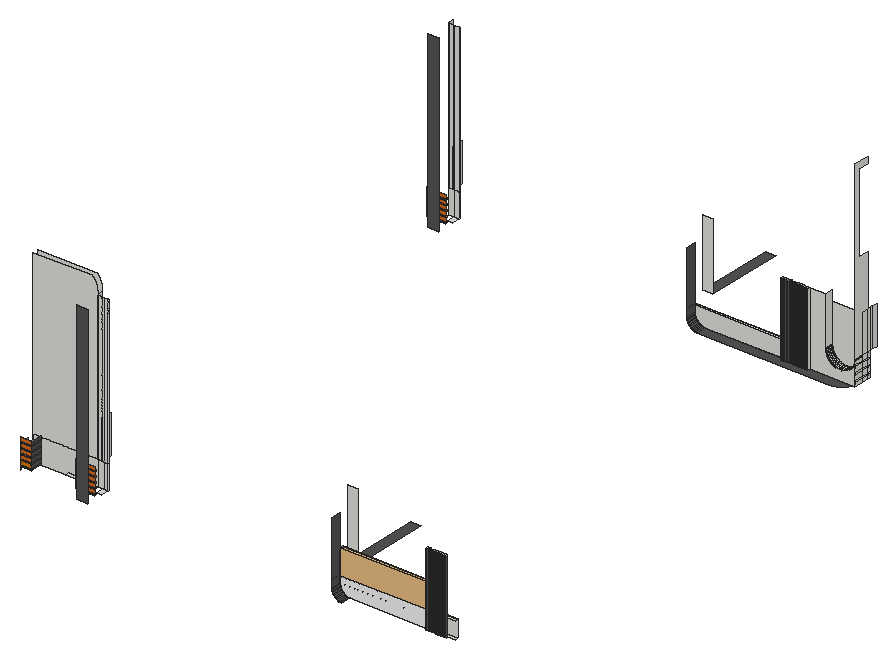
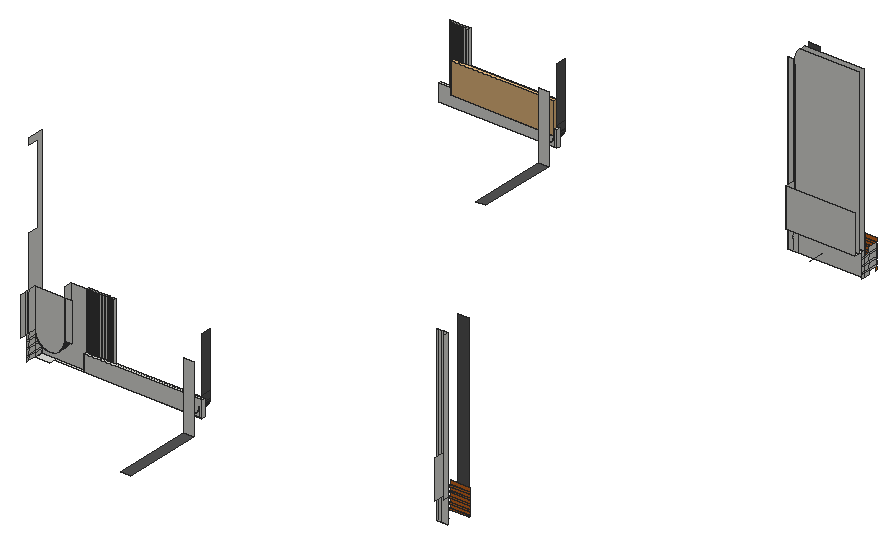
# SketchUp Ruby script. Lengths in inches.
U = 1.inch
M = Sketchup.active_model
def pt(a) = Geom::Point3d.new(a.map { |v| v * U })
def face(e, loops, mat)
  f = e.add_face(loops[0].map { |a| pt(a) })
  loops[1..].each { |l| e.add_face(l.map { |a| pt(a) }).erase! }
  f.material = f.back_material = mat if mat
  f
end
# faces: each face lists its corners as indices into pts; further lists are holes
def faces(e, pts, list, mat = nil) = list.each { |f| face(e, (f[0].is_a?(Array) ? f : [f]).map { |l| l.map { |i| pts[i] } }, mat) }
# xy, xz, yz: faces in a plane at the given z, y or x. An outline is a flat list of corners, or four numbers for a rectangle; further outlines are holes
def ring(l) = l.size == 4 ? [[l[0], l[1]], [l[2], l[1]], [l[2], l[3]], [l[0], l[3]]] : l.each_slice(2).to_a
def flat(e, list, mat, &to3) = list.each { |f| face(e, (f[0].is_a?(Array) ? f : [f]).map { |l| ring(l).map { |u, v| to3.(u, v) } }, mat) }
def xy(e, z, list, mat = nil) = flat(e, list, mat) { |x, y| [x, y, z] }
def xz(e, y, list, mat = nil) = flat(e, list, mat) { |x, z| [x, y, z] }
def yz(e, x, list, mat = nil) = flat(e, list, mat) { |y, z| [x, y, z] }
def lines(e, pts, list) = list.each { |a, b| e.add_line(pt(pts[a]), pt(pts[b])) }
# prism: a flat outline (further loops are holes) pulled along v
def prism(e, loops, v, mat = nil)
  f = face(e, loops, mat); d = Geom::Vector3d.new(v.map { |x| x * U })
  f.pushpull(f.normal.samedirection?(d) ? d.length : -d.length)
end
def box(e, o, s, mat = nil) = prism(e, [[o, [o[0] + s[0], o[1], o[2]], [o[0] + s[0], o[1] + s[1], o[2]], [o[0], o[1] + s[1], o[2]]]], [0, 0, s[2]], mat)
def at(x, y, z, deg = 0) = Geom::Transformation.translation(pt([x, y, z])) * Geom::Transformation.rotation(ORIGIN, Z_AXIS, deg.degrees)
def axes(o, x, y, z) = Geom::Transformation.new([*x, 0, *y, 0, *z, 0, *pt(o).to_a, 1])
def part(name) = M.definitions.add(name)
# library, detail: a bought-in or finely detailed component or shape, given as its bounding box
def library(name, o, s) = part(name).tap { |d| box(d.entities, o, s) }
def detail(e, o, s) = box(e.add_group.entities, o, s)
def put(e, d, t, mat = nil) = e.add_instance(d, t).tap { |i| i.material = mat if mat }
def group(e, t, mat = nil) = e.add_group.tap { |g| g.transformation = t; g.material = mat if mat }.entities
root = M.entities
M.materials.add("[0039_DarkOrange]").color = [219, 120, 0]
M.materials.add("[0041_Chocolate]").color = [210, 105, 30]
M.materials.add("[0129_WhiteSmoke]").color = [245, 245, 245]
M.materials.add("[Color M06]").color = [84, 84, 84]
c1 = library("Glass Railing",[0,0,0],[139.5,4.76,42])
xy(root,141.26,[[1326.04,281.47,1343.48,285.84],[1343.48,281.47,1486.5,285.84],[991.85,292.45,998.64,302.46],[1254.35,972.36,1271.79,976.74],[1271.79,972.36,1414.82,976.74],
  [1414.82,972.36,1455.4,976.74],[1455.4,972.36,1473.39,972.36,1474.14,973.89,1475.18,976.95,1475.8125,980.12,1476.02,983.34,1455.4,983.34],[1473.39,972.36,1474.14,973.89,1475.18,976.95,1475.8125,980.12,1476.02,983.34,1476.02,972.36],[915.16,983.34,921.96,993.35]])
xy(root,141.26,[[1271.79,958.64,1451.32,958.64,1454.55,958.86,1457.72,959.49,1460.78,960.52,1463.67,961.95,1466.36,963.75,1468.79,965.88,1470.92,968.31,1472.71,970.99,1473.39,972.36,1414.82,972.36,1414.82,969.24,1411.69,969.24,1411.69,972.36,1410.44,972.36,1410.44,969.24,1407.32,969.24,1407.32,972.36,1406.25,972.36,1406.25,969.24,1403.13,969.24,1403.13,972.36,1402.07,972.36,1402.07,969.24,1398.94,969.24,1398.94,972.36,1397.88,972.36,1397.88,969.24,1394.75,969.24,1394.75,972.36,1393.69,972.36,1393.69,969.24,1390.57,969.24,1390.57,972.36,1389.44,972.36,1389.44,969.24,1386.32,969.24,1386.32,972.36,1385.19,972.36,1385.19,969.24,1382.07,969.24,1382.07,972.36,1380.94,972.36,1380.94,969.24,1377.82,969.24,1377.82,972.36,1271.79,972.36]],"[Color M06]")
xy(root,145.27,[[946.98,295.65,972.17,300.34]])
xy(root,145.27,[[897.21,280.47,912.6,281.47]],"[0039_DarkOrange]")
xy(root,145.27,[[972.17,280.47,998.64,281.47],[895.48,971.36,921.96,972.36]],"[0041_Chocolate]")
xy(root,147.375,[[897.21,280.47,912.6,281.47]],"[0039_DarkOrange]")
xy(root,147.375,[[972.17,280.47,998.64,281.47],[895.48,971.36,921.96,972.36]],"[0041_Chocolate]")
xy(root,148.66,[[1299.4,333.33,1313.11,439.98],[1227.71,1024.22,1241.43,1130.875]],"[Color M06]")
xy(root,152.33,[[897.21,280.47,912.6,281.47]],"[0039_DarkOrange]")
xy(root,152.33,[[972.17,280.47,998.64,281.47],[895.48,971.36,921.96,972.36]],"[0041_Chocolate]")
xy(root,154.4375,[[897.21,280.47,912.6,281.47],[972.17,280.47,998.64,281.47],[895.48,971.36,921.96,972.36]],"[0041_Chocolate]")
xy(root,159.39,[[897.21,280.47,912.6,281.47],[972.17,280.47,998.64,281.47],[895.48,971.36,921.96,972.36]],"[0041_Chocolate]")
xy(root,161.5,[[897.21,280.47,912.6,281.47],[972.17,280.47,998.64,281.47],[895.48,971.36,921.96,972.36]],"[0041_Chocolate]")
xy(root,163.7,[[1326.04,281.47,1343.48,285.84],[1343.48,281.47,1486.5,285.84],[1254.35,972.36,1271.79,976.74],[1271.79,972.36,1414.82,976.74]])
xy(root,166.45,[[897.21,280.47,912.6,281.47],[972.17,280.47,998.64,281.47],[895.48,971.36,921.96,972.36]],"[0041_Chocolate]")
xy(root,168.5625,[[897.21,280.47,912.6,281.47],[972.17,280.47,998.64,281.47],[895.48,971.36,921.96,972.36]],"[0041_Chocolate]")
xy(root,173.52,[[897.21,280.47,912.6,281.47],[972.17,280.47,998.64,281.47],[895.48,971.36,921.96,972.36]],"[0041_Chocolate]")
xy(root,174.51,[[897.21,302.46,984.18,310.27],[984.18,302.46,984.18,310.27,897.21,310.27,897.21,317.3125,990.02,317.3125,990.02,302.46]])
xy(root,175.625,[[897.21,280.47,912.6,281.47],[972.17,280.47,998.64,281.47],[895.48,971.36,921.96,972.36]],"[0041_Chocolate]")
xz(root,267.75,[[984.18,141.3,999.52,376.875]],"[Color M06]")
xz(root,278.34,[[1449.5,141.26,1452.63,240.16],[1453.75,141.26,1456.88,240.16],[1458,141.26,1461.13,240.16],[1462.25,141.26,1465.38,240.16],[1466.44,141.26,1469.57,240.16],
  [1470.63,141.26,1473.75,240.16],[1474.82,141.26,1477.94,240.16]],"[Color M06]")
xz(root,280.47,[[897.21,147.375,912.6,152.33]],"[0039_DarkOrange]")
xz(root,280.47,[[972.17,147.375,998.64,152.33],[897.21,154.4375,912.6,159.39],[972.17,154.4375,998.64,159.39],[897.21,161.5,912.6,166.45],[972.17,161.5,998.64,166.45],
  [897.21,168.5625,912.6,173.52],[972.17,168.5625,998.64,173.52],[897.21,175.625,912.6,180.58],[972.17,175.625,998.64,180.58]],"[0041_Chocolate]")
xz(root,281.47,[[1326.04,141.26,1330.04,163.7],[1330.04,141.26,1343.48,141.26,1341.7,141.46,1339.96,141.89,1338.29,142.53,1336.71,143.38,1335.25,144.42,1333.93,145.64,1332.78,147.01,1331.82,148.52,1331.05,150.14,1330.49,151.84,1330.15,153.6,1330.04,155.39],[1449.5,141.26,1452.63,163.7],[1452.63,141.26,1453.75,163.7],[1453.75,141.26,1456.88,163.7],
  [1456.88,141.26,1458,163.7],[1458,141.26,1461.13,163.7],[1461.13,141.26,1462.25,163.7],[1462.25,141.26,1465.38,163.7],[1465.38,141.26,1466.44,163.7],
  [1466.44,141.26,1469.57,163.7],[1469.57,141.26,1470.63,163.7],[1470.63,141.26,1473.75,163.7],[1473.75,141.26,1474.82,163.7],[1449.5,163.7,1452.63,240.16],
  [1453.75,163.7,1456.88,240.16],[1458,163.7,1461.13,240.16],[1462.25,163.7,1465.38,240.16],[1466.44,163.7,1469.57,240.16],[1470.63,163.7,1473.75,240.16]])
xz(root,281.47,[[897.21,145.27,912.6,147.375]],"[0039_DarkOrange]")
xz(root,281.47,[[972.17,145.27,998.64,147.375],[897.21,152.33,912.6,154.4375],[972.17,152.33,998.64,154.4375],[897.21,159.39,912.6,161.5],[972.17,159.39,998.64,161.5],
  [897.21,166.45,912.6,168.5625],[972.17,166.45,998.64,168.5625],[897.21,173.52,912.6,175.625],[972.17,173.52,998.64,175.625]],"[0041_Chocolate]")
xz(root,281.47,[[1343.48,141.26,1449.5,141.26,1449.5,163.7,1330.04,163.7,1330.04,155.39,1330.15,153.6,1330.49,151.84,1331.05,150.14,1331.82,148.52,1332.78,147.01,1333.93,145.64,1335.25,144.42,1336.71,143.38,1338.29,142.53,1339.96,141.89,1341.7,141.46]],"[0129_WhiteSmoke]")
xz(root,285.84,[[1326.04,141.26,1326.04,163.7,1343.48,163.7,1343.48,141.26,1341.7,141.46,1339.96,141.89,1338.29,142.53,1336.71,143.38,1335.25,144.42,1333.93,145.64,1332.78,147.01,1331.82,148.52,1331.05,150.14,1330.49,151.84,1330.15,153.6,1330.04,155.39,1330.04,141.26],[1330.04,141.26,1330.04,155.39,1330.15,153.6,1330.49,151.84,1331.05,150.14,1331.82,148.52,1332.78,147.01,1333.93,145.64,1335.25,144.42,1336.71,143.38,1338.29,142.53,1339.96,141.89,1341.7,141.46,1343.48,141.26],[1343.48,141.26,1486.5,163.7]])
xz(root,302.46,[[897.21,141.26,984.18,174.51],[984.18,141.26,992.73,174.51],[992.73,141.26,998.64,174.51],[998.64,141.26,999.52,174.51],[897.21,174.51,984.18,174.51,984.18,376.875,984.17,377.55,984.14,378.22,984.1,378.9,984.04,379.57,983.96,380.24,983.86,380.9,983.75,381.57,983.62,382.23,983.47,382.89,983.3,383.54,983.28,383.64,983.12,384.19,982.92,384.84,982.7,385.47,982.6,385.76,982.47,386.11,982.22,386.73,981.95,387.35,981.67,387.96,981.37,388.57,981.06,389.17,980.73,389.76,980.38,390.33,980.02,390.9,979.65,391.47,979.26,392.02,978.86,392.56,978.4375,393.09,978.4,393.14,978.01,393.6,977.5625,394.11,977.1,394.61,976.63,395.09,976.46,395.26,897.21,395.26],
  [984.18,174.51,990.02,374.14],[990.02,174.51,992.73,374.14],[992.73,174.51,998.64,374.14],[998.64,174.51,999.52,374.14]])
xz(root,310.27,[[897.21,174.51,897.21,395.26,976.46,395.26,976.63,395.09,977.1,394.61,977.5625,394.11,978.01,393.6,978.4,393.14,978.4375,393.09,978.86,392.56,979.26,392.02,979.65,391.47,980.02,390.9,980.38,390.33,980.73,389.76,981.06,389.17,981.37,388.57,981.67,387.96,981.95,387.35,982.22,386.73,982.47,386.11,982.6,385.76,982.7,385.47,982.92,384.84,983.12,384.19,983.28,383.64,983.3,383.54,983.47,382.89,983.62,382.23,983.75,381.57,983.86,380.9,983.96,380.24,984.04,379.57,984.1,378.9,984.14,378.22,984.17,377.55,984.18,376.875,984.18,174.51]])
xz(root,317.3125,[[897.21,174.51,990.02,226.8]])
xz(root,333.33,[[1299.4,148.66,1313.11,240.16]])
xz(root,958.64,[[907.49,141.3,922.83,376.875]],"[Color M06]")
xz(root,969.24,[[1377.82,141.26,1380.94,240.16],[1382.07,141.26,1385.19,240.16],[1386.32,141.26,1389.44,240.16],[1390.57,141.26,1393.69,240.16],[1394.75,141.26,1397.88,240.16],
  [1398.94,141.26,1402.07,240.16],[1403.13,141.26,1406.25,240.16],[1407.32,141.26,1410.44,240.16],[1411.69,141.26,1414.82,240.16]],"[Color M06]")
xz(root,971.36,[[895.48,147.375,921.96,152.33],[895.48,154.4375,921.96,159.39],[895.48,161.5,921.96,166.45],[895.48,168.5625,921.96,173.52],[895.48,175.625,921.96,180.58]],"[0041_Chocolate]")
xz(root,972.36,[[1254.35,141.26,1258.35,163.7],[1258.35,141.26,1271.79,141.26,1270.01,141.46,1268.27,141.89,1266.6,142.53,1265.02,143.38,1263.5625,144.42,1262.25,145.64,1261.1,147.01,1260.13,148.52,1259.36,150.14,1258.8,151.84,1258.46,153.6,1258.35,155.39],[1271.79,141.26,1377.82,141.26,1377.82,163.7,1258.35,163.7,1258.35,155.39,1258.46,153.6,1258.8,151.84,1259.36,150.14,1260.13,148.52,1261.1,147.01,1262.25,145.64,1263.5625,144.42,1265.02,143.38,1266.6,142.53,1268.27,141.89,1270.01,141.46],[1377.82,141.26,1380.94,163.7],[1380.94,141.26,1382.07,163.7],
  [1382.07,141.26,1385.19,163.7],[1385.19,141.26,1386.32,163.7],[1386.32,141.26,1389.44,163.7],[1389.44,141.26,1390.57,163.7],[1390.57,141.26,1393.69,163.7],
  [1393.69,141.26,1394.75,163.7],[1394.75,141.26,1397.88,163.7],[1397.88,141.26,1398.94,163.7],[1398.94,141.26,1402.07,163.7],[1402.07,141.26,1403.13,163.7],
  [1403.13,141.26,1406.25,163.7],[1406.25,141.26,1407.32,163.7],[1407.32,141.26,1410.44,163.7],[1410.44,141.26,1411.69,163.7],[1411.69,141.26,1414.82,163.7],
  [1414.82,141.26,1476.02,141.26,1476.02,174.51,1476,173.46,1475.91,172.42,1475.78,171.38,1475.59,170.36,1475.34,169.34,1475.05,168.33,1474.7,167.35,1474.3,166.38,1473.85,165.4375,1473.35,164.52,1472.8,163.625,1472.21,162.76,1471.57,161.93,1470.89,161.14,1470.17,160.38,1469.41,159.66,1468.62,158.98,1467.79,158.34,1466.92,157.75,1466.03,157.2,1465.11,156.7,1464.17,156.25,1463.2,155.85,1462.21,155.5,1461.21,155.21,1460.19,154.96,1459.17,154.77,1458.13,154.64,1457.09,154.55,1456.04,154.53,1454.99,154.55,1453.95,154.64,1452.91,154.77,1451.88,154.96,1450.87,155.21,1449.86,155.5,1448.88,155.85,1447.91,156.25,1446.97,156.7,1446.05,157.2,1445.16,157.75,1444.29,158.34,1443.46,158.98,1442.67,159.66,1441.91,160.38,1441.1875,161.14,1440.51,161.93,1439.87,162.76,1439.28,163.625,1438.73,164.52,1438.23,165.4375,1437.78,166.38,1437.38,167.35,1437.03,168.33,1436.74,169.34,1436.49,170.36,1436.3,171.38,1436.16,172.42,1436.08,173.46,1436.06,174.51,1436.06,240.16,1414.82,240.16],[1377.82,163.7,1380.94,240.16],[1382.07,163.7,1385.19,240.16],[1386.32,163.7,1389.44,240.16],[1390.57,163.7,1393.69,240.16],
  [1394.75,163.7,1397.88,240.16],[1398.94,163.7,1402.07,240.16],[1403.13,163.7,1406.25,240.16],[1407.32,163.7,1410.44,240.16],[1411.69,163.7,1414.82,240.16]])
xz(root,972.36,[[895.48,145.27,921.96,147.375],[895.48,152.33,921.96,154.4375],[895.48,159.39,921.96,161.5],[895.48,166.45,921.96,168.5625],[895.48,173.52,921.96,175.625]],"[0041_Chocolate]")
xz(root,976.74,[[1254.35,141.26,1254.35,163.7,1271.79,163.7,1271.79,141.26,1270.01,141.46,1268.27,141.89,1266.6,142.53,1265.02,143.38,1263.5625,144.42,1262.25,145.64,1261.1,147.01,1260.13,148.52,1259.36,150.14,1258.8,151.84,1258.46,153.6,1258.35,155.39,1258.35,141.26],[1258.35,141.26,1258.35,155.39,1258.46,153.6,1258.8,151.84,1259.36,150.14,1260.13,148.52,1261.1,147.01,1262.25,145.64,1263.5625,144.42,1265.02,143.38,1266.6,142.53,1268.27,141.89,1270.01,141.46,1271.79,141.26],[1271.79,141.26,1414.82,163.7]])
xz(root,983.34,[[1456.04,154.53,1457.09,154.55,1458.13,154.64,1459.17,154.77,1460.19,154.96,1461.21,155.21,1462.21,155.5,1463.2,155.85,1464.17,156.25,1465.11,156.7,1466.03,157.2,1466.92,157.75,1467.79,158.34,1468.62,158.98,1469.41,159.66,1470.17,160.38,1470.89,161.14,1471.57,161.93,1472.21,162.76,1472.8,163.625,1473.35,164.52,1473.85,165.4375,1474.3,166.38,1474.7,167.35,1475.05,168.33,1475.34,169.34,1475.59,170.36,1475.78,171.38,1475.91,172.42,1476,173.46,1476.02,174.51,1476.02,226.8,1436.06,226.8,1436.06,174.51,1436.08,173.46,1436.16,172.42,1436.3,171.38,1436.49,170.36,1436.74,169.34,1437.03,168.33,1437.38,167.35,1437.78,166.38,1438.23,165.4375,1438.73,164.52,1439.28,163.625,1439.87,162.76,1440.51,161.93,1441.1875,161.14,1441.91,160.38,1442.67,159.66,1443.46,158.98,1444.29,158.34,1445.16,157.75,1446.05,157.2,1446.97,156.7,1447.91,156.25,1448.88,155.85,1449.86,155.5,1450.87,155.21,1451.88,154.96,1452.91,154.77,1453.95,154.64,1454.99,154.55],[1426.4,174.51,1436.06,226.8]])
xz(root,993.35,[[907.49,141.26,916.04,174.51],[916.04,141.26,921.96,174.51],[921.96,141.26,922.83,174.51],[907.49,174.51,913.34,374.14],[913.34,174.51,916.04,374.14],
  [916.04,174.51,921.96,374.14],[921.96,174.51,922.83,374.14]])
xz(root,1024.22,[[1227.71,148.66,1241.43,240.16]])
yz(root,897.21,[[292.45,141.26,302.46,146.14],[302.46,141.26,305.58,146.14],[281.47,146.14,292.45,148.26],[292.45,146.14,302.46,148.26],[302.46,146.14,305.58,148.26],
  [281.47,148.26,292.45,155.64],[292.45,148.26,302.46,155.64],[302.46,148.26,305.58,155.64],[281.47,155.64,292.45,157.76],[292.45,155.64,302.46,157.76],
  [302.46,155.64,305.58,157.76],[281.47,157.76,292.45,165.14],[292.45,157.76,302.46,165.14],[302.46,157.76,305.58,165.14],[281.47,165.14,292.45,167.26],
  [292.45,165.14,302.46,167.26],[302.46,165.14,305.58,167.26],[281.47,167.26,292.45,174.51],[302.46,167.26,305.58,174.51]])
yz(root,897.21,[[280.47,141.26,281.47,145.27],[280.47,147.375,281.47,148.26],[280.47,148.26,281.47,152.33]],"[0039_DarkOrange]")
yz(root,897.21,[[280.47,154.4375,281.47,155.64],[280.47,155.64,281.47,157.76],[280.47,157.76,281.47,159.39],[280.47,161.5,281.47,165.14],[280.47,165.14,281.47,166.45],
  [280.47,168.5625,281.47,173.52]],"[0041_Chocolate]")
yz(root,907.49,[[993.35,174.51,1001.16,374.14]])
yz(root,912.6,[[281.47,145.27,295.65,147.375],[280.47,147.375,295.65,152.33],[281.47,152.33,295.65,154.4375],[280.47,154.4375,295.65,159.39],[281.47,159.39,295.65,161.5],
  [280.47,161.5,295.65,166.45],[281.47,166.45,295.65,168.5625],[280.47,168.5625,295.65,173.52],[281.47,173.52,295.65,175.625],[280.47,175.625,295.65,180.58]],"[Color M06]")
yz(root,913.34,[[993.35,174.51,1008.21,226.8]])
yz(root,972.17,[[281.47,145.27,295.65,147.375],[280.47,147.375,295.65,152.33],[281.47,152.33,295.65,154.4375],[280.47,154.4375,295.65,159.39],[281.47,159.39,295.65,161.5],
  [280.47,161.5,295.65,166.45],[281.47,166.45,295.65,168.5625],[280.47,168.5625,295.65,173.52],[281.47,173.52,295.65,175.625],[280.47,175.625,295.65,180.58]],"[Color M06]")
yz(root,984.18,[[302.46,174.51,310.27,374.14]])
yz(root,990.02,[[302.46,174.51,317.3125,226.8]])
yz(root,1254.35,[[972.36,141.26,976.74,163.7]])
yz(root,1258.35,[[958.64,155.39,972.36,164.97],[958.64,164.97,972.36,240.16]],"[Color M06]")
yz(root,1326.04,[[281.47,141.26,285.84,163.7]])
yz(root,1330.04,[[267.75,155.39,281.47,164.97],[267.75,164.97,281.47,240.16]],"[Color M06]")
yz(root,1377.82,[[969.24,141.26,972.36,240.16]])
yz(root,1380.94,[[969.24,141.26,972.36,240.16]])
yz(root,1382.07,[[969.24,141.26,972.36,240.16]])
yz(root,1385.19,[[969.24,141.26,972.36,240.16]])
yz(root,1386.32,[[969.24,141.26,972.36,240.16]])
yz(root,1389.44,[[969.24,141.26,972.36,240.16]])
yz(root,1390.57,[[969.24,141.26,972.36,240.16]])
yz(root,1393.69,[[969.24,141.26,972.36,240.16]])
yz(root,1394.75,[[969.24,141.26,972.36,240.16]])
yz(root,1397.88,[[969.24,141.26,972.36,240.16]])
yz(root,1398.94,[[969.24,141.26,972.36,240.16]])
yz(root,1402.07,[[969.24,141.26,972.36,240.16]])
yz(root,1403.13,[[969.24,141.26,972.36,240.16]])
yz(root,1406.25,[[969.24,141.26,972.36,240.16]])
yz(root,1407.32,[[969.24,141.26,972.36,240.16]])
yz(root,1410.44,[[969.24,141.26,972.36,240.16]])
yz(root,1411.69,[[969.24,141.26,972.36,240.16]])
yz(root,1414.82,[[969.24,141.26,972.36,240.16],[972.36,141.26,976.74,163.7]])
yz(root,1436.06,[[972.36,174.51,983.34,240.16]])
yz(root,1449.5,[[278.34,141.26,281.47,240.16]])
yz(root,1452.63,[[278.34,141.26,281.47,240.16]])
yz(root,1453.75,[[278.34,141.26,281.47,240.16]])
yz(root,1456.88,[[278.34,141.26,281.47,240.16]])
yz(root,1458,[[278.34,141.26,281.47,240.16]])
yz(root,1461.13,[[278.34,141.26,281.47,240.16]])
yz(root,1462.25,[[278.34,141.26,281.47,240.16]])
yz(root,1465.38,[[278.34,141.26,281.47,240.16]])
yz(root,1466.44,[[278.34,141.26,281.47,240.16]])
yz(root,1469.57,[[278.34,141.26,281.47,240.16]])
yz(root,1470.63,[[278.34,141.26,281.47,240.16]])
yz(root,1473.75,[[278.34,141.26,281.47,240.16]])
yz(root,1474.82,[[278.34,141.26,281.47,240.16]])
yz(root,1476.02,[[972.36,141.26,983.34,146.14],[983.34,141.26,993.35,146.14],[993.35,141.26,996.48,146.14],[972.36,146.14,983.34,148.26],[983.34,146.14,993.35,148.26],
  [993.35,146.14,996.48,148.26],[972.36,148.26,983.34,155.64],[983.34,148.26,993.35,155.64],[993.35,148.26,996.48,155.64],[972.36,155.64,983.34,157.76],
  [983.34,155.64,993.35,157.76],[993.35,155.64,996.48,157.76],[972.36,157.76,983.34,165.14],[983.34,157.76,993.35,165.14],[993.35,157.76,996.48,165.14],
  [972.36,165.14,983.34,167.26],[983.34,165.14,993.35,167.26],[993.35,165.14,996.48,167.26],[972.36,167.26,983.34,174.51],[983.34,167.26,993.35,174.51],
  [993.35,167.26,996.48,174.51],[972.36,174.51,972.36,175.625,971.36,175.625,971.36,180.58,972.36,180.58,972.36,182.6875,971.36,182.6875,971.36,187.64,972.36,187.64,972.36,189.75,971.36,189.75,971.36,194.7,972.36,194.7,972.36,196.8125,971.36,196.8125,971.36,201.77,972.36,201.77,972.36,203.875,971.36,203.875,971.36,208.83,972.36,208.83,972.36,210.9375,971.36,210.9375,971.36,215.89,972.36,215.89,972.36,218,971.36,218,971.36,222.95,972.36,222.95,972.36,225.0625,971.36,225.0625,971.36,230.02,972.36,230.02,972.36,232.125,971.36,232.125,971.36,237.08,972.36,237.08,972.36,239.1875,971.36,239.1875,971.36,244.14,972.36,244.14,972.36,246.25,971.36,246.25,971.36,251.2,972.36,251.2,972.36,253.3125,971.36,253.3125,971.36,258.27,972.36,258.27,972.36,260.375,971.36,260.375,971.36,265.33,972.36,265.33,972.36,267.4375,971.36,267.4375,971.36,272.39,972.36,272.39,972.36,274.5,971.36,274.5,971.36,279.45,972.36,279.45,972.36,281.5625,971.36,281.5625,971.36,286.52,972.36,286.52,972.36,288.625,971.36,288.625,971.36,293.58,972.36,293.58,972.36,295.6875,971.36,295.6875,971.36,300.64,972.36,300.64,972.36,302.75,971.36,302.75,971.36,307.7,972.36,307.7,972.36,309.8125,971.36,309.8125,971.36,314.77,972.36,314.77,972.36,316.875,971.36,316.875,971.36,321.83,972.36,321.83,972.36,323.9375,971.36,323.9375,971.36,328.89,972.36,328.89,972.36,331,971.36,331,971.36,335.95,972.36,335.95,972.36,338.0625,971.36,338.0625,971.36,343.02,972.36,343.02,972.36,345.125,971.36,345.125,971.36,350.08,972.36,350.08,972.36,352.1875,971.36,352.1875,971.36,357.14,972.36,357.14,972.36,359.25,971.36,359.25,971.36,364.2,972.36,364.2,972.36,366.3125,971.36,366.3125,971.36,371.27,972.36,371.27,972.36,373.1875,971.36,373.1875,971.36,378.14,972.36,378.14,972.36,380.0625,971.36,380.0625,971.36,385.02,972.36,385.02,972.36,386.9375,971.36,386.9375,971.36,391.89,972.36,391.89,972.36,393.8125,971.36,393.8125,971.36,398.77,972.36,398.77,972.36,400.6875,971.36,400.6875,971.36,405.64,972.36,405.64,972.36,411.82,993.35,411.82,993.35,402.64,978.84,402.64,978.84,295.72,992.96,295.72,992.96,226.8,983.34,226.8,983.34,174.51],[983.34,174.51,993.35,226.8],[993.35,174.51,996.48,226.8],[996.48,174.51,1001.16,226.8],
  [1001.16,174.51,1008.21,226.8]])
yz(root,1476.02,[[971.36,141.26,972.36,145.27],[971.36,147.375,972.36,148.26],[971.36,148.26,972.36,152.33]],"[0039_DarkOrange]")
yz(root,1476.02,[[971.36,154.4375,972.36,155.64],[971.36,155.64,972.36,157.76],[971.36,157.76,972.36,159.39],[971.36,161.5,972.36,165.14],[971.36,165.14,972.36,166.45],
  [971.36,168.5625,972.36,173.52]],"[0041_Chocolate]")
p = [[1341.7,267.75,141.46],[1343.48,267.75,141.26],[1343.48,281.47,141.26],[1341.7,281.47,141.46],[1343.48,285.84,141.26],[1341.7,285.84,141.46],
  [1270.01,958.64,141.46],[1271.79,958.64,141.26],[1271.79,972.36,141.26],[1270.01,972.36,141.46],[1271.79,976.74,141.26],[1270.01,976.74,141.46],
  [1339.96,267.75,141.89],[1339.96,281.47,141.89],[1339.96,285.84,141.89],[1268.27,958.64,141.89],[1268.27,972.36,141.89],[1268.27,976.74,141.89],
  [1338.29,267.75,142.53],[1338.29,281.47,142.53],[1338.29,285.84,142.53],[1266.6,958.64,142.53],[1266.6,972.36,142.53],[1266.6,976.74,142.53],
  [1336.71,267.75,143.38],[1336.71,281.47,143.38],[1336.71,285.84,143.38],[1265.02,958.64,143.38],[1265.02,972.36,143.38],[1265.02,976.74,143.38],
  [1335.25,267.75,144.42],[1335.25,281.47,144.42],[1335.25,285.84,144.42],[1263.5625,958.64,144.42],[1263.5625,972.36,144.42],[1263.5625,976.74,144.42],
  [1333.93,267.75,145.64],[1333.93,281.47,145.64],[1333.93,285.84,145.64],[1262.25,958.64,145.64],[1262.25,972.36,145.64],[1262.25,976.74,145.64],
  [1332.78,267.75,147.01],[1332.78,281.47,147.01],[1332.78,285.84,147.01],[1261.1,958.64,147.01],[1261.1,972.36,147.01],[1261.1,976.74,147.01],
  [1331.82,267.75,148.52],[1331.82,281.47,148.52],[1331.82,285.84,148.52],[1260.13,958.64,148.52],[1260.13,972.36,148.52],[1260.13,976.74,148.52],
  [1331.05,267.75,150.14],[1331.05,281.47,150.14],[1331.05,285.84,150.14],[1259.36,958.64,150.14],[1259.36,972.36,150.14],[1259.36,976.74,150.14],
  [1330.49,267.75,151.84],[1330.49,281.47,151.84],[1330.49,285.84,151.84],[1258.8,958.64,151.84],[1258.8,972.36,151.84],[1258.8,976.74,151.84],
  [1330.15,267.75,153.6],[1330.15,281.47,153.6],[1330.15,285.84,153.6],[1258.46,958.64,153.6],[1258.46,972.36,153.6],[1258.46,976.74,153.6],
  [1330.04,267.75,155.39],[1330.04,281.47,155.39],[1330.04,285.84,155.39],[1258.35,958.64,155.39],[1258.35,972.36,155.39],[1258.35,976.74,155.39],
  [1456.04,983.34,154.53],[1454.99,983.34,154.55],[1454.99,972.36,154.55],[1456.04,972.36,154.53],[1457.09,983.34,154.55],[1457.09,972.36,154.55],
  [1453.95,983.34,154.64],[1452.91,983.34,154.77],[1452.91,972.36,154.77],[1453.95,972.36,154.64],[1458.13,983.34,154.64],[1458.13,972.36,154.64],
  [1459.17,983.34,154.77],[1459.17,972.36,154.77],[1451.88,983.34,154.96],[1451.88,972.36,154.96],[1460.19,983.34,154.96],[1460.19,972.36,154.96],
  [1450.87,983.34,155.21],[1450.87,972.36,155.21],[1461.21,983.34,155.21],[1461.21,972.36,155.21],[1449.86,983.34,155.5],[1449.86,972.36,155.5],
  [1462.21,983.34,155.5],[1462.21,972.36,155.5],[1448.88,983.34,155.85],[1448.88,972.36,155.85],[1463.2,983.34,155.85],[1463.2,972.36,155.85],
  [1447.91,983.34,156.25],[1447.91,972.36,156.25],[1464.17,983.34,156.25],[1464.17,972.36,156.25],[1446.97,983.34,156.7],[1446.97,972.36,156.7],
  [1465.11,983.34,156.7],[1465.11,972.36,156.7],[1446.05,983.34,157.2],[1446.05,972.36,157.2],[1466.03,983.34,157.2],[1466.03,972.36,157.2],
  [1445.16,983.34,157.75],[1445.16,972.36,157.75],[1466.92,983.34,157.75],[1466.92,972.36,157.75],[1444.29,983.34,158.34],[1444.29,972.36,158.34],
  [1467.79,983.34,158.34],[1467.79,972.36,158.34],[1443.46,983.34,158.98],[1443.46,972.36,158.98],[1468.62,983.34,158.98],[1468.62,972.36,158.98],
  [1442.67,983.34,159.66],[1442.67,972.36,159.66],[1469.41,983.34,159.66],[1469.41,972.36,159.66],[1441.91,983.34,160.38],[1441.91,972.36,160.38],
  [1470.17,983.34,160.38],[1470.17,972.36,160.38],[1441.1875,983.34,161.14],[1441.1875,972.36,161.14],[1470.89,983.34,161.14],[1470.89,972.36,161.14],
  [1440.51,983.34,161.93],[1440.51,972.36,161.93],[1471.57,983.34,161.93],[1471.57,972.36,161.93],[1439.87,983.34,162.76],[1439.87,972.36,162.76],
  [1472.21,983.34,162.76],[1472.21,972.36,162.76],[1439.28,983.34,163.625],[1439.28,972.36,163.625],[1472.8,983.34,163.625],[1472.8,972.36,163.625],
  [1438.73,983.34,164.52],[1438.73,972.36,164.52],[1473.35,983.34,164.52],[1473.35,972.36,164.52],[1438.23,983.34,165.4375],[1438.23,972.36,165.4375],
  [1473.85,983.34,165.4375],[1473.85,972.36,165.4375],[1437.78,983.34,166.38],[1437.78,972.36,166.38],[1474.3,983.34,166.38],[1474.3,972.36,166.38],
  [1437.38,983.34,167.35],[1437.38,972.36,167.35],[1474.7,983.34,167.35],[1474.7,972.36,167.35],[1437.03,983.34,168.33],[1437.03,972.36,168.33],
  [1475.05,983.34,168.33],[1475.05,972.36,168.33],[1436.74,983.34,169.34],[1436.74,972.36,169.34],[1475.34,983.34,169.34],[1475.34,972.36,169.34],
  [1436.49,983.34,170.36],[1436.49,972.36,170.36],[1475.59,983.34,170.36],[1475.59,972.36,170.36],[1436.3,983.34,171.38],[1436.3,972.36,171.38],
  [1475.78,983.34,171.38],[1475.78,972.36,171.38],[1436.16,983.34,172.42],[1436.16,972.36,172.42],[1475.91,983.34,172.42],[1475.91,972.36,172.42],
  [1436.08,983.34,173.46],[1436.08,972.36,173.46],[1476,983.34,173.46],[1476,972.36,173.46],[1436.06,983.34,174.51],[1436.06,972.36,174.51],
  [1476.02,983.34,174.51],[1476.02,972.36,174.51],[937.76,321.34,165.14],[937.76,343.15,165.14]]
faces(root,p,[[0,1,2,3],[6,7,8,9],[12,0,3,13],[15,6,9,16],[18,12,13,19],[21,15,16,22],[24,18,19,25],[27,21,22,28],
  [30,24,25,31],[33,27,28,34],[36,30,31,37],[39,33,34,40],[42,36,37,43],[45,39,40,46],[48,42,43,49],[51,45,46,52],
  [54,48,49,55],[57,51,52,58],[60,54,55,61],[63,57,58,64],[66,60,61,67],[69,63,64,70],[72,66,67,73],[75,69,70,76]],"[Color M06]")
faces(root,p,[[3,2,4,5],[9,8,10,11],[13,3,5,14],[16,9,11,17],[19,13,14,20],[22,16,17,23],[25,19,20,26],[28,22,23,29],
  [31,25,26,32],[34,28,29,35],[37,31,32,38],[40,34,35,41],[43,37,38,44],[46,40,41,47],[49,43,44,50],[52,46,47,53],
  [55,49,50,56],[58,52,53,59],[61,55,56,62],[64,58,59,65],[67,61,62,68],[70,64,65,71],[73,67,68,74],[76,70,71,77],
  [78,79,80,81],[82,78,81,83],[84,85,86,87],[79,84,87,80],[88,82,83,89],[90,88,89,91],[85,92,93,86],[94,90,91,95],
  [92,96,97,93],[98,94,95,99],[96,100,101,97],[102,98,99,103],[100,104,105,101],[106,102,103,107],[104,108,109,105],[110,106,107,111],
  [108,112,113,109],[114,110,111,115],[112,116,117,113],[118,114,115,119],[116,120,121,117],[122,118,119,123],[120,124,125,121],[126,122,123,127],
  [124,128,129,125],[130,126,127,131],[128,132,133,129],[134,130,131,135],[132,136,137,133],[138,134,135,139],[136,140,141,137],[142,138,139,143],
  [140,144,145,141],[146,142,143,147],[144,148,149,145],[150,146,147,151],[148,152,153,149],[154,150,151,155],[152,156,157,153],[158,154,155,159],
  [156,160,161,157],[162,158,159,163],[160,164,165,161],[166,162,163,167],[164,168,169,165],[170,166,167,171],[168,172,173,169],[174,170,171,175],
  [172,176,177,173],[178,174,175,179],[176,180,181,177],[182,178,179,183],[180,184,185,181],[186,182,183,187],[184,188,189,185],[190,186,187,191],
  [188,192,193,189],[194,190,191,195],[192,196,197,193],[198,194,195,199]])
lines(root,p,[[200,201]])
put(root,c1,at(1330.04,281.47,155.39))
